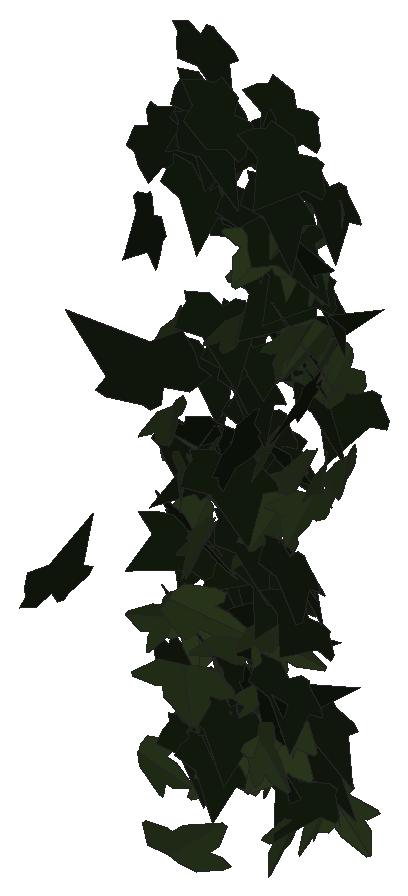
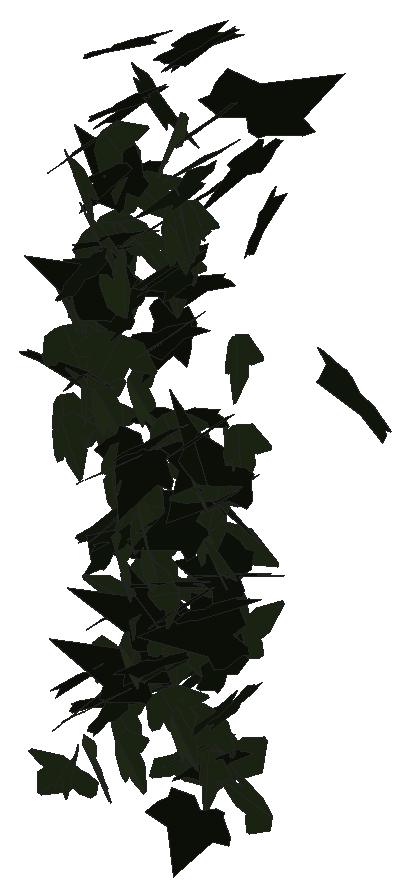
# SketchUp Ruby script. Lengths in inches.
U = 1.inch
M = Sketchup.active_model
def pt(a) = Geom::Point3d.new(a.map { |v| v * U })
def face(e, loops, mat)
  f = e.add_face(loops[0].map { |a| pt(a) })
  loops[1..].each { |l| e.add_face(l.map { |a| pt(a) }).erase! }
  f.material = f.back_material = mat if mat
  f
end
# faces: each face lists its corners as indices into pts; further lists are holes
def faces(e, pts, list, mat = nil) = list.each { |f| face(e, (f[0].is_a?(Array) ? f : [f]).map { |l| l.map { |i| pts[i] } }, mat) }
# xy, xz, yz: faces in a plane at the given z, y or x. An outline is a flat list of corners, or four numbers for a rectangle; further outlines are holes
def ring(l) = l.size == 4 ? [[l[0], l[1]], [l[2], l[1]], [l[2], l[3]], [l[0], l[3]]] : l.each_slice(2).to_a
def flat(e, list, mat, &to3) = list.each { |f| face(e, (f[0].is_a?(Array) ? f : [f]).map { |l| ring(l).map { |u, v| to3.(u, v) } }, mat) }
def xy(e, z, list, mat = nil) = flat(e, list, mat) { |x, y| [x, y, z] }
def xz(e, y, list, mat = nil) = flat(e, list, mat) { |x, z| [x, y, z] }
def yz(e, x, list, mat = nil) = flat(e, list, mat) { |y, z| [x, y, z] }
def lines(e, pts, list) = list.each { |a, b| e.add_line(pt(pts[a]), pt(pts[b])) }
# prism: a flat outline (further loops are holes) pulled along v
def prism(e, loops, v, mat = nil)
  f = face(e, loops, mat); d = Geom::Vector3d.new(v.map { |x| x * U })
  f.pushpull(f.normal.samedirection?(d) ? d.length : -d.length)
end
def box(e, o, s, mat = nil) = prism(e, [[o, [o[0] + s[0], o[1], o[2]], [o[0] + s[0], o[1] + s[1], o[2]], [o[0], o[1] + s[1], o[2]]]], [0, 0, s[2]], mat)
def at(x, y, z, deg = 0) = Geom::Transformation.translation(pt([x, y, z])) * Geom::Transformation.rotation(ORIGIN, Z_AXIS, deg.degrees)
def axes(o, x, y, z) = Geom::Transformation.new([*x, 0, *y, 0, *z, 0, *pt(o).to_a, 1])
def part(name) = M.definitions.add(name)
# library, detail: a bought-in or finely detailed component or shape, given as its bounding box
def library(name, o, s) = part(name).tap { |d| box(d.entities, o, s) }
def detail(e, o, s) = box(e.add_group.entities, o, s)
def put(e, d, t, mat = nil) = e.add_instance(d, t).tap { |i| i.material = mat if mat }
def group(e, t, mat = nil) = e.add_group.tap { |g| g.transformation = t; g.material = mat if mat }.entities
root = M.entities
M.materials.add("1026 AP 7946 SUNNY SIDE UP").color = [254, 231, 186]
M.materials.add("efeu1").color = [18, 25, 13]
M.materials.add("efeu2").color = [43, 57, 29]
c1 = part("ivyleaf_9")
p = [[1.54,2.16,1.25],[1.36,2.04,1.19],[-0.21,0.99,0.68],[-0.71,1.11,0.82],[-0.85,0.86,0.67],[-0.8,0.17,0.21],
  [-0.9,-0.01,0.1],[-0.67,-0.16,-0.02],[-0.08,-0.08,-0.05],[-0.03,-0.6,-0.4],[0.65,-0.88,-0.66],[0.83,-0.6,-0.49],
  [1.29,-0.42,-0.43],[1.8125,-0.07,-0.26],[1.21,0.44,0.15]]
faces(c1.entities,p,[[0,1,2,3,4,5,6,7,8,9,10,11,12,13,14]],"efeu1")
c2 = part("ivyleaf_10")
p = [[0,0.5,-0.03],[-0.0625,2.02,-0.43],[-0.19,2.01,-0.46],[-0.54,1.05,-0.29],[-0.52,0.625,-0.18],[-0.83,0.76,-0.28],
  [-1.16,0.64,-0.33],[-1.15,0.33,-0.24],[-0.77,-0.39,0.02],[-0.3,-0.51,0.16],[0.04,-0.48,0.23],[-0.02,2.01,-0.4375],
  [-0.06,2.01,-0.43],[0.04,-0.49,0.23],[0.67,-0.49,0.14],[1.38,0.36,-0.2],[1.375,0.51,-0.24],[0.81,0.65,-0.19],
  [0.62,0.59,-0.15],[0.6,1.09,-0.28],[0.5,1.23,-0.31]]
faces(c2.entities,p,[[0,1,2,3,4,5,6,7,8,9,10],[11,12,0,13,14,15,16,17,18,19,20]],"efeu2")
put(root,c1,axes([114.58,212.84,282.9],[-0.22038,-0.28928,0.05312],[-0.01341,-0.05491,-0.33106],[0.4623,-0.13949,0.01572]),"1026 AP 7946 SUNNY SIDE UP")
put(root,c1,axes([114.5,211.84,289.67],[0.21549,-0.17371,-0.32569],[-0.19839,0.29264,-0.22098],[0.52993,0.18019,0.04971]),"1026 AP 7946 SUNNY SIDE UP")
put(root,c2,axes([114.73,211.9375,282.02],[-0.07728,-0.11998,-0.35255],[-0.21039,-0.31424,0.13172],[-0.52889,0.14253,-0.00089]),"1026 AP 7946 SUNNY SIDE UP")
put(root,c2,axes([114.29,212.12,279.56],[-0.01905,-0.02116,-0.34342],[0.39995,-0.21662,0.00338],[-0.34016,-0.25351,0.02321]),"1026 AP 7946 SUNNY SIDE UP")
put(root,c2,axes([114.67,212.03,285.18],[-0.06831,-0.33084,-0.06862],[0.03714,0.06211,-0.34304],[0.52878,-0.0471,0.01523]),"1026 AP 7946 SUNNY SIDE UP")
put(root,c1,axes([114.65,212.98,279.74],[0.41387,0.11395,-0.11655],[-0.18573,-0.01156,-0.29349],[-0.1721,0.28651,0.03646]),"1026 AP 7946 SUNNY SIDE UP")
put(root,c1,axes([114.45,212.35,281.24],[0.21928,-0.28954,-0.04148],[-0.01302,0.03886,-0.33071],[0.45912,0.13939,0.01043]),"1026 AP 7946 SUNNY SIDE UP")
put(root,c2,axes([114.71,212.03,286.5625],[0.00107,-0.3309,-0.09887],[0.05564,0.09366,-0.33851],[0.53807,-0.00903,0.0352]),"1026 AP 7946 SUNNY SIDE UP")
put(root,c1,axes([114.49,212.98,290.6],[0.12598,-0.34085,-0.01581],[0.00994,0.01526,-0.36049],[0.53628,0.07979,0.0104]),"1026 AP 7946 SUNNY SIDE UP")
put(root,c1,axes([114.88,212.31,283.09],[-0.42051,-0.13326,0.14679],[-0.08895,-0.17958,-0.28195],[0.29449,-0.24452,0.12444]),"1026 AP 7946 SUNNY SIDE UP")
put(root,c1,axes([114.49,212.39,284.58],[0.27882,-0.24816,-0.14559],[-0.02167,0.15714,-0.3042],[0.44743,0.16225,0.076]),"1026 AP 7946 SUNNY SIDE UP")
put(root,c1,axes([114.36,212.67,282.51],[0.43636,-0.0205,0.1783],[0.2721,-0.00808,-0.28669],[0.03408,0.32702,0.00602]),"1026 AP 7946 SUNNY SIDE UP")
put(root,c1,axes([114.63,211.6875,288.39],[0.09069,-0.16293,-0.33434],[0.35294,-0.24117,0.16489],[-0.44723,-0.22337,0.06233]),"1026 AP 7946 SUNNY SIDE UP")
put(root,c2,axes([114.68,212.53,284.54],[0.33463,0.26404,0.01542],[0.03471,-0.00052,-0.3489],[-0.41426,0.21324,-0.01678]),"1026 AP 7946 SUNNY SIDE UP")
put(root,c1,axes([114.43,212.43,283.3],[0.3313,-0.1951,0.18166],[0.17265,-0.1416,-0.29553],[0.37703,0.23628,-0.02429]),"1026 AP 7946 SUNNY SIDE UP")
put(root,c1,axes([114.66,212.91,285.63],[0.02258,-0.32972,0.04131],[0.0011,-0.04198,-0.34025],[0.52264,0.01434,-0.00107]),"1026 AP 7946 SUNNY SIDE UP")
put(root,c2,axes([114.85,212.47,280.21],[0.01746,-0.29293,-0.13535],[0.04285,0.13019,-0.29971],[0.50192,-0.00093,0.03029]),"1026 AP 7946 SUNNY SIDE UP")
put(root,c1,axes([114.5625,212.5,281.77],[0.10135,-0.21569,0.23287],[0.15687,-0.20583,-0.23159],[0.46704,0.11594,0.02725]),"1026 AP 7946 SUNNY SIDE UP")
put(root,c2,axes([114.88,212.43,283.57],[0.40016,-0.21378,0.02821],[0.0047,-0.04072,-0.34132],[0.33911,0.25283,-0.02855]),"1026 AP 7946 SUNNY SIDE UP")
put(root,c1,axes([114.75,212.33,284.85],[0.47498,0.1731,0.01553],[0.04236,-0.01876,-0.35747],[-0.26977,0.30182,-0.02878]),"1026 AP 7946 SUNNY SIDE UP")
put(root,c2,axes([114.91,212.95,289.11],[0.37554,-0.2474,-0.04236],[0.01544,0.06407,-0.34993],[0.39369,0.23348,0.05413]),"1026 AP 7946 SUNNY SIDE UP")
put(root,c2,axes([115.02,212.94,288.66],[-0.02352,-0.34098,0.04456],[0.00001,-0.04524,-0.35188],[0.54085,-0.01483,0.00194]),"1026 AP 7946 SUNNY SIDE UP")
put(root,c1,axes([115.21,212.23,284.43],[-0.44513,0.16165,-0.08893],[0.09109,-0.07354,-0.33444],[-0.2741,-0.28696,0.03328]),"1026 AP 7946 SUNNY SIDE UP")
put(root,c2,axes([115.09,212.76,288.86],[-0.13165,-0.32957,-0.06683],[0.02391,0.06114,-0.34995],[0.52706,-0.08509,-0.00082]),"1026 AP 7946 SUNNY SIDE UP")
put(root,c1,axes([114.78,212.85,289.51],[0.35689,-0.23602,-0.12388],[-0.0478,0.13238,-0.32971],[0.41279,0.21938,0.06892]),"1026 AP 7946 SUNNY SIDE UP")
put(root,c2,axes([114.97,212.28,281.93],[0.39915,0.2432,-0.00787],[0.0169,-0.02423,-0.36139],[-0.38229,0.25285,-0.0242]),"1026 AP 7946 SUNNY SIDE UP")
put(root,c2,axes([115.1,212.44,284.63],[0.19923,-0.28799,0.12221],[0.03803,-0.12035,-0.32384],[0.48926,0.12662,-0.02459]),"1026 AP 7946 SUNNY SIDE UP")
put(root,c1,axes([115,212.29,280.1],[-0.09276,-0.32021,-0.00661],[0.01114,0.00337,-0.33534],[0.50342,-0.05907,0.0062]),"1026 AP 7946 SUNNY SIDE UP")
put(root,c1,axes([114.83,212.96,288.18],[0.333,-0.269,0.00824],[0.02476,0.00028,-0.35246],[0.42251,0.21199,0.01416]),"1026 AP 7946 SUNNY SIDE UP")
put(root,c1,axes([115,212.92,282.82],[0.0096,-0.3209,0.03841],[0.00361,-0.03906,-0.33088],[0.50831,0.00634,0.00162]),"1026 AP 7946 SUNNY SIDE UP")
put(root,c1,axes([115.04,212.5625,289.57],[-0.1124,-0.31457,0.15233],[0.01649,-0.15464,-0.33063],[0.54751,-0.05992,0.04123]),"1026 AP 7946 SUNNY SIDE UP")
put(root,c1,axes([115.03,212.375,284.77],[0.07041,0.29212,0.19621],[-0.07295,-0.18364,0.30298],[0.54203,-0.06266,0.01529]),"1026 AP 7946 SUNNY SIDE UP")
put(root,c1,axes([115.01,212.29,280.77],[0.04606,-0.29826,0.11801],[0.02103,-0.11549,-0.30941],[0.50291,0.03215,0.00213]),"1026 AP 7946 SUNNY SIDE UP")
put(root,c2,axes([115.23,212.67,280.74],[0.11797,-0.3036,0.07875],[0.01699,-0.07782,-0.32253],[0.49266,0.07538,-0.00773]),"1026 AP 7946 SUNNY SIDE UP")
put(root,c1,axes([115.03,212.96,288.16],[0.13532,-0.31905,-0.09319],[-0.0073,0.09042,-0.33937],[0.52062,0.08419,0.01947]),"1026 AP 7946 SUNNY SIDE UP")
put(root,c2,axes([115.3,212,283.47],[0.0343,-0.3366,0.04549],[-0.00179,-0.04624,-0.34774],[0.5342,0.02146,-0.00409]),"1026 AP 7946 SUNNY SIDE UP")
put(root,c1,axes([114.97,212.69,284.07],[0.4748,-0.1437,0.01439],[0.00109,-0.03282,-0.34337],[0.22715,0.30054,-0.02843]),"1026 AP 7946 SUNNY SIDE UP")
put(root,c2,axes([115.3125,211.49,284.67],[0.23852,-0.25697,-0.16286],[-0.01421,0.17143,-0.29776],[0.47298,0.13474,0.07318]),"1026 AP 7946 SUNNY SIDE UP")
put(root,c1,axes([115.16,212.08,288.93],[-0.04166,-0.3328,0.11502],[-0.01963,-0.1129,-0.34458],[0.55257,-0.0291,-0.00357]),"1026 AP 7946 SUNNY SIDE UP")
put(root,c1,axes([115.375,208.59,284.14],[-0.39717,0.32181,-0.12292],[-0.08975,0.10899,0.42151],[0.53317,0.25807,-0.02061]),"1026 AP 7946 SUNNY SIDE UP")
put(root,c2,axes([115.1875,212.23,284.39],[-0.45676,0.08372,-0.15354],[0.18754,-0.1125,-0.30428],[-0.19346,-0.30672,0.06753]),"1026 AP 7946 SUNNY SIDE UP")
put(root,c2,axes([115.26,212.0625,280.59],[-0.51709,0.07722,-0.08909],[0.12058,-0.05193,-0.34674],[-0.13742,-0.33616,0.03099]),"1026 AP 7946 SUNNY SIDE UP")
put(root,c2,axes([115.44,212.65,281.0625],[-0.1905,-0.27005,0.13265],[-0.0037,-0.13967,-0.30129],[0.47145,-0.11021,0.05123]),"1026 AP 7946 SUNNY SIDE UP")
put(root,c2,axes([115.1875,212.94,283.01],[-0.21967,0.16431,-0.24736],[0.20804,-0.2025,-0.22239],[-0.40881,-0.19135,0.01974]),"1026 AP 7946 SUNNY SIDE UP")
put(root,c1,axes([115.57,212.8125,282.93],[-0.38924,-0.17642,0.11532],[-0.04013,-0.14814,-0.29688],[0.32693,-0.22823,0.10086]),"1026 AP 7946 SUNNY SIDE UP")
put(root,c2,axes([115.41,212.43,289.98],[0.24308,-0.25212,-0.21234],[0.11922,0.24845,-0.25482],[0.49652,0.06378,0.16514]),"1026 AP 7946 SUNNY SIDE UP")
put(root,c2,axes([115.57,212.2,279.92],[0.34474,0.14864,-0.20121],[-0.22389,-0.13766,-0.27222],[-0.31564,0.25999,-0.02666]),"1026 AP 7946 SUNNY SIDE UP")
put(root,c2,axes([115.47,211.82,283.71],[0.12165,-0.28523,0.20019],[0.07665,-0.18979,-0.30557],[0.5387,0.09142,-0.00173]),"1026 AP 7946 SUNNY SIDE UP")
put(root,c1,axes([115.46,212.08,280.02],[-0.09676,-0.30982,0.07186],[0.01044,-0.07408,-0.32516],[0.49986,-0.05842,0.0207]),"1026 AP 7946 SUNNY SIDE UP")
put(root,c2,axes([115.625,212.2,281.82],[-0.28215,-0.26977,-0.02776],[0.04586,0.01108,-0.3332],[0.42359,-0.18089,0.01758]),"1026 AP 7946 SUNNY SIDE UP")
put(root,c2,axes([115.24,211.7,282.48],[-0.1766,-0.07564,-0.33362],[0.51651,0.02522,-0.12345],[0.07728,-0.34143,0.06269]),"1026 AP 7946 SUNNY SIDE UP")
put(root,c2,axes([115.67,212.68,283.27],[0.01768,-0.30032,0.14059],[-0.00036,-0.13826,-0.31038],[0.51981,0.01012,-0.005]),"1026 AP 7946 SUNNY SIDE UP")
put(root,c1,axes([115.42,212.29,281.08],[0.1957,-0.29002,-0.01198],[0.00225,0.01147,-0.325],[0.45629,0.12433,0.00674]),"1026 AP 7946 SUNNY SIDE UP")
put(root,c1,axes([115.64,212.49,286.6],[-0.10076,-0.29176,0.17125],[-0.03286,-0.16712,-0.3084],[0.52827,-0.06605,0.01348]),"1026 AP 7946 SUNNY SIDE UP")
put(root,c1,axes([115.55,212.79,281.72],[0.00188,-0.30727,-0.09968],[0.06674,0.09433,-0.31318],[0.5013,-0.0114,0.04207]),"1026 AP 7946 SUNNY SIDE UP")
put(root,c1,axes([115.67,212.88,285.13],[-0.10425,-0.31558,0.08094],[-0.00105,-0.08187,-0.33229],[0.51205,-0.06442,0.0158]),"1026 AP 7946 SUNNY SIDE UP")
put(root,c1,axes([115.64,212.66,288.46],[-0.01061,-0.33982,0.07516],[0.00772,-0.07498,-0.35053],[0.5471,-0.00553,0.00641]),"1026 AP 7946 SUNNY SIDE UP")
put(root,c1,axes([115.72,212.4,281.36],[-0.14728,-0.24713,0.19154],[0.03181,-0.20014,-0.26275],[0.48657,-0.06172,0.07515]),"1026 AP 7946 SUNNY SIDE UP")
put(root,c1,axes([115.7,211.91,287.2],[-0.13045,-0.32526,-0.09243],[0.0624,0.08044,-0.34484],[0.52608,-0.09019,0.01798]),"1026 AP 7946 SUNNY SIDE UP")
put(root,c2,axes([115.89,212.6,283.73],[0.14154,-0.31567,-0.05351],[-0.00775,0.05072,-0.33774],[0.50252,0.08969,0.00986]),"1026 AP 7946 SUNNY SIDE UP")
put(root,c1,axes([115.67,212.43,282.125],[-0.22308,0.19174,0.24342],[0.23533,-0.18165,0.24449],[0.41507,0.20603,-0.00779]),"1026 AP 7946 SUNNY SIDE UP")
put(root,c1,axes([115.7,211.63,290.77],[0.00157,-0.3656,0.01363],[-0.00124,-0.01531,-0.37673],[0.57538,0.00097,-0.00085]),"1026 AP 7946 SUNNY SIDE UP")
put(root,c1,axes([115.93,212.18,280.9],[-0.27549,-0.17461,0.25612],[-0.09371,-0.26273,-0.23398],[0.46972,-0.15482,0.10353]),"1026 AP 7946 SUNNY SIDE UP")
put(root,c1,axes([115.85,212.27,280.63],[-0.09645,0.01977,0.33532],[-0.04787,-0.32999,0.01281],[0.51033,-0.02722,0.06458]),"1026 AP 7946 SUNNY SIDE UP")
put(root,c2,axes([116,211.91,284.83],[-0.12862,-0.32027,0.07906],[0.00526,-0.08175,-0.34019],[0.51849,-0.07862,0.02307]),"1026 AP 7946 SUNNY SIDE UP")
put(root,c1,axes([115.9,212.61,284.78],[0.46673,0.02472,-0.16165],[-0.24289,-0.03385,-0.30645],[-0.05915,0.3341,-0.0171]),"1026 AP 7946 SUNNY SIDE UP")
put(root,c1,axes([115.8,212.28,283.68],[0.05575,-0.33782,-0.03487],[-0.00761,0.0316,-0.34974],[0.5335,0.03575,-0.00134]),"1026 AP 7946 SUNNY SIDE UP")
put(root,c2,axes([115.8,210.85,279.1875],[-0.43923,-0.15837,0.20532],[0.27643,0.09583,0.33135],[-0.29103,0.33004,0.00486]),"1026 AP 7946 SUNNY SIDE UP")
put(root,c1,axes([115.93,212.27,286.49],[-0.18511,-0.31883,-0.03189],[0.02306,0.02565,-0.34994],[0.50289,-0.11854,0.00431]),"1026 AP 7946 SUNNY SIDE UP")
put(root,c2,axes([116.01,212.48,283.59],[-0.03589,-0.30003,0.12337],[0.08891,-0.12358,-0.30427],[0.50112,0.00044,0.06282]),"1026 AP 7946 SUNNY SIDE UP")
put(root,c1,axes([116.14,211.54,290.59],[-0.27042,-0.2164,0.26198],[-0.2138,-0.21738,-0.2852],[0.48116,-0.21821,0.02051]),"1026 AP 7946 SUNNY SIDE UP")
put(root,c2,axes([116.32,212.29,287.91],[0.34714,-0.1433,-0.25196],[-0.36297,0.08728,-0.26772],[0.25679,0.31708,-0.0378]),"1026 AP 7946 SUNNY SIDE UP")
put(root,c2,axes([116.14,211.67,287.28],[-0.07439,-0.34948,-0.04904],[0.01822,0.04446,-0.36301],[0.55388,-0.0484,0.00536]),"1026 AP 7946 SUNNY SIDE UP")
put(root,c1,axes([115.84,212.79,284.84],[0.2303,-0.26888,-0.13905],[0.03417,0.1576,-0.30162],[0.47076,0.1201,0.08992]),"1026 AP 7946 SUNNY SIDE UP")
put(root,c2,axes([116.13,212.49,283.47],[0.26643,-0.28288,0.04833],[0.00795,-0.0534,-0.33919],[0.45123,0.16797,-0.02256]),"1026 AP 7946 SUNNY SIDE UP")
put(root,c2,axes([116.12,212.43,284.16],[-0.12245,-0.26821,-0.19946],[0.12294,0.17675,-0.28585],[0.50396,-0.10828,0.02127]),"1026 AP 7946 SUNNY SIDE UP")
put(root,c1,axes([116.02,211.69,284.94],[-0.18233,-0.29627,-0.14831],[0.10751,0.12583,-0.32659],[0.50548,-0.13363,0.01597]),"1026 AP 7946 SUNNY SIDE UP")
put(root,c2,axes([116.21,212.62,280.03],[0.06433,-0.3097,0.07393],[-0.00042,-0.07416,-0.3221],[0.5005,0.03974,-0.00978]),"1026 AP 7946 SUNNY SIDE UP")
put(root,c2,axes([116.22,212.76,283.22],[0.17121,-0.30566,-0.05483],[-0.02033,0.05004,-0.33395],[0.48697,0.10956,0.00533]),"1026 AP 7946 SUNNY SIDE UP")
put(root,c1,axes([115.76,212.25,281.9],[0.14453,0.02541,0.35255],[0.53309,-0.06053,-0.08958],[0.08194,0.34899,-0.03909]),"1026 AP 7946 SUNNY SIDE UP")
put(root,c1,axes([116.36,212.03,290.13],[-0.42947,0.16175,-0.16575],[0.183,-0.11873,-0.32533],[-0.30973,-0.29442,0.03761]),"1026 AP 7946 SUNNY SIDE UP")
put(root,c1,axes([115.98,211.19,290.5],[0.10536,-0.34869,-0.04692],[0.00165,0.04455,-0.3654],[0.55253,0.06635,0.01004]),"1026 AP 7946 SUNNY SIDE UP")
put(root,c1,axes([116.02,212.15,286.23],[0.02462,-0.34362,0.06673],[0.01343,-0.0664,-0.35471],[0.55024,0.017,0.00567]),"1026 AP 7946 SUNNY SIDE UP")
put(root,c1,axes([116.12,211.54,281.22],[-0.16106,-0.33639,0.00899],[0.00916,-0.01289,-0.36221],[0.52913,-0.10217,0.00901]),"1026 AP 7946 SUNNY SIDE UP")
put(root,c2,axes([116.18,212.59,281.53],[0.16795,-0.25146,0.17375],[0.09534,-0.159,-0.28233],[0.46774,0.1227,-0.00484]),"1026 AP 7946 SUNNY SIDE UP")
put(root,c2,axes([116.35,212.35,284.15],[-0.25227,-0.2762,0.17514],[-0.05062,-0.17689,-0.3254],[0.50875,-0.15455,0.05447]),"1026 AP 7946 SUNNY SIDE UP")
put(root,c2,axes([116.3,210.37,282.34],[-0.58209,-0.15484,-0.01178],[0.03674,-0.0286,-0.41194],[0.24125,-0.36923,0.0343]),"1026 AP 7946 SUNNY SIDE UP")
put(root,c1,axes([116.25,212.79,290.17],[-0.22223,-0.27482,0.17472],[-0.06742,-0.16923,-0.31738],[0.5046,-0.14364,0.03454]),"1026 AP 7946 SUNNY SIDE UP")
put(root,c2,axes([116.3,212.48,284.54],[-0.18727,-0.2919,-0.09384],[0.05974,0.08107,-0.32428],[0.47631,-0.12493,0.00378]),"1026 AP 7946 SUNNY SIDE UP")
put(root,c2,axes([116.33,212.04,281.65],[0.00404,0.18807,-0.28793],[0.02051,0.28031,0.19533],[0.5307,-0.01227,-0.00536]),"1026 AP 7946 SUNNY SIDE UP")
put(root,c2,axes([116.36,211.95,281.37],[-0.01427,-0.274,0.18412],[0.04764,-0.18028,-0.28176],[0.51353,0.00911,0.03126]),"1026 AP 7946 SUNNY SIDE UP")
put(root,c2,axes([116.49,211.98,288.46],[-0.32963,-0.17098,0.23159],[-0.07498,-0.25558,-0.2465],[0.43897,-0.17205,0.1318]),"1026 AP 7946 SUNNY SIDE UP")
put(root,c2,axes([116.32,212.71,286.34],[-0.40872,-0.19956,-0.10814],[0.18936,0.01059,-0.33146],[0.29877,-0.27971,0.06213]),"1026 AP 7946 SUNNY SIDE UP")
put(root,c2,axes([116.375,211.96,282.45],[-0.13446,-0.2698,-0.17854],[0.11763,0.156,-0.28988],[0.48896,-0.11172,0.02064]),"1026 AP 7946 SUNNY SIDE UP")
put(root,c2,axes([116.44,212.08,285.35],[0.14124,-0.30955,0.12017],[0.03757,-0.11631,-0.3326],[0.51977,0.09252,-0.00861]),"1026 AP 7946 SUNNY SIDE UP")
put(root,c2,axes([116.37,212.5,286.92],[-0.039,-0.27475,-0.22374],[0.03567,-0.21698,0.28087],[-0.54801,0.00543,0.0342]),"1026 AP 7946 SUNNY SIDE UP")
put(root,c1,axes([116.5,212.35,283.05],[-0.2915,-0.25978,0.05256],[-0.03074,-0.05049,-0.32879],[0.4156,-0.18594,0.01255]),"1026 AP 7946 SUNNY SIDE UP")
put(root,c1,axes([116.14,212.3,280.99],[0.08505,-0.00661,0.36191],[0.54936,0.03907,-0.05442],[-0.05915,0.35332,0.01488]),"1026 AP 7946 SUNNY SIDE UP")
put(root,c1,axes([116.59,212.27,287.6],[-0.36354,-0.22439,0.14805],[-0.03558,-0.1746,-0.31658],[0.41857,-0.20973,0.10167]),"1026 AP 7946 SUNNY SIDE UP")
put(root,c1,axes([116.24,212.49,286.85],[0.3027,-0.26109,0.10857],[0.07245,-0.09854,-0.3341],[0.43764,0.1969,-0.01978]),"1026 AP 7946 SUNNY SIDE UP")
put(root,c1,axes([116.36,212.72,283.13],[0.11816,-0.27756,0.16679],[0.07314,-0.15675,-0.29713],[0.50119,0.08831,0.00404]),"1026 AP 7946 SUNNY SIDE UP")
put(root,c1,axes([116.67,212.57,287.83],[-0.32635,-0.24641,0.12373],[-0.04549,-0.13182,-0.32711],[0.4296,-0.20115,0.05935]),"1026 AP 7946 SUNNY SIDE UP")
put(root,c1,axes([116.73,210.87,285.89],[-0.03286,0.0321,-0.41799],[-0.38491,0.32382,0.04126],[0.51166,0.24566,0.00419]),"1026 AP 7946 SUNNY SIDE UP")
put(root,c1,axes([116.43,211.84,281.18],[-0.07393,0.01427,0.34833],[0.17853,-0.32084,0.02834],[0.50116,0.11639,0.04129]),"1026 AP 7946 SUNNY SIDE UP")
put(root,c2,axes([116.26,212.23,282.08],[-0.01998,0.03127,0.36672],[0.56156,-0.0034,0.01343],[0.00712,0.356,-0.02999]),"1026 AP 7946 SUNNY SIDE UP")
put(root,c1,axes([116.56,212.31,283.41],[0.03901,-0.32786,0.08158],[-0.00972,-0.08169,-0.33898],[0.53096,0.02259,-0.0122]),"1026 AP 7946 SUNNY SIDE UP")
put(root,c1,axes([117.13,208.74,287.95],[0.08011,0.08408,0.43915],[-0.6809,-0.01915,0.05716],[0.04615,-0.42841,0.08102]),"1026 AP 7946 SUNNY SIDE UP")
put(root,c1,axes([116.59,212.05,288.73],[0.04839,-0.2835,-0.22652],[0.02183,0.21986,-0.29088],[0.56217,0.01587,0.0308]),"1026 AP 7946 SUNNY SIDE UP")
put(root,c2,axes([116.77,211.97,281.04],[0.5185,-0.08056,-0.00787],[-0.02248,-0.0284,-0.3484],[0.12518,0.3286,-0.02999]),"1026 AP 7946 SUNNY SIDE UP")
put(root,c2,axes([116.86,211.71,280.77],[0.31992,0.20166,-0.19645],[-0.18059,-0.15563,-0.29493],[-0.39865,0.23233,-0.02405]),"1026 AP 7946 SUNNY SIDE UP")
put(root,c2,axes([116.88,212.07,289.08],[-0.09087,-0.29389,0.18029],[0.01049,-0.18009,-0.30743],[0.53908,-0.04603,0.03637]),"1026 AP 7946 SUNNY SIDE UP")
put(root,c1,axes([116.73,212.32,280.21],[-0.08043,-0.20406,0.2667],[0.01585,-0.26398,-0.21291],[0.51952,-0.02354,0.04779]),"1026 AP 7946 SUNNY SIDE UP")
put(root,c1,axes([116.83,212.71,280.47],[-0.18895,-0.24172,0.17538],[-0.03646,-0.17695,-0.27451],[0.4647,-0.11217,0.04977]),"1026 AP 7946 SUNNY SIDE UP")
put(root,c2,axes([116.87,212.48,287.97],[0.40478,-0.23718,-0.0007],[-0.02603,-0.01895,-0.35978],[0.37203,0.25673,-0.02441]),"1026 AP 7946 SUNNY SIDE UP")
put(root,c1,axes([116.68,212.73,285.96],[0.14581,-0.31725,0.03971],[0.00433,-0.04121,-0.34062],[0.50284,0.09235,-0.00858]),"1026 AP 7946 SUNNY SIDE UP")
put(root,c2,axes([116.91,212.25,285.11],[0.07058,-0.30802,0.15098],[0.05187,-0.14498,-0.32133],[0.53504,0.05468,0.01123]),"1026 AP 7946 SUNNY SIDE UP")
put(root,c1,axes([116.69,212.93,287.38],[0.08394,-0.2851,0.1834],[0.06751,-0.17465,-0.2997],[0.52554,0.06797,0.00921]),"1026 AP 7946 SUNNY SIDE UP")
put(root,c1,axes([116.62,212.41,286.86],[0.06679,-0.04284,0.36121],[0.53214,0.10695,-0.02813],[-0.16045,0.33686,0.05707]),"1026 AP 7946 SUNNY SIDE UP")
put(root,c2,axes([116.93,212.89,279.7],[-0.09585,0.30429,-0.03479],[-0.03146,-0.04007,-0.3187],[-0.48068,-0.05805,0.0278]),"1026 AP 7946 SUNNY SIDE UP")
put(root,c2,axes([117.06,212.79,286.24],[-0.27035,-0.277,0.09396],[-0.03205,-0.09602,-0.3348],[0.45822,-0.17015,0.03202]),"1026 AP 7946 SUNNY SIDE UP")
put(root,c2,axes([117,212.71,288.88],[0.36084,-0.25076,-0.06437],[-0.04825,0.05461,-0.34956],[0.40294,0.2311,0.01579]),"1026 AP 7946 SUNNY SIDE UP")
put(root,c2,axes([117,212.5625,286.79],[-0.01178,-0.30962,0.1459],[0.04016,-0.14352,-0.31875],[0.53502,0.00396,0.02714]),"1026 AP 7946 SUNNY SIDE UP")
put(root,c1,axes([116.83,211.96,281.73],[-0.05061,-0.33824,0.09066],[0.00128,-0.09038,-0.35043],[0.55032,-0.03089,0.00915]),"1026 AP 7946 SUNNY SIDE UP")
put(root,c1,axes([116.64,212.125,288.43],[0.06356,-0.09599,0.35124],[0.27375,-0.29409,-0.10811],[0.48597,0.17822,0.01496]),"1026 AP 7946 SUNNY SIDE UP")
put(root,c2,axes([117.01,212.36,279.54],[0.28582,-0.27742,0.02795],[-0.00001,-0.03427,-0.34134],[0.43855,0.18081,-0.01823]),"1026 AP 7946 SUNNY SIDE UP")
put(root,c1,axes([116.83,211.73,289.51],[0.00063,-0.35463,0.02047],[0.00361,-0.02189,-0.36545],[0.55867,0.00054,0.00234]),"1026 AP 7946 SUNNY SIDE UP")
put(root,c2,axes([117.09,212.8,284.79],[-0.02438,-0.33108,0.03681],[0.00745,-0.03787,-0.3416],[0.52388,-0.01487,0.00657]),"1026 AP 7946 SUNNY SIDE UP")
put(root,c2,axes([117.13,212,284.625],[-0.19897,-0.29288,0.11724],[-0.01812,-0.12005,-0.32742],[0.49469,-0.1222,0.03516]),"1026 AP 7946 SUNNY SIDE UP")
put(root,c1,axes([116.74,212.15,287.17],[0.22358,-0.24814,0.19229],[0.12674,-0.17037,-0.29535],[0.47289,0.16298,-0.01176]),"1026 AP 7946 SUNNY SIDE UP")
put(root,c1,axes([116.91,212.56,280.97],[0.06678,-0.30995,-0.07842],[0.02017,0.07662,-0.32101],[0.50079,0.03824,0.02339]),"1026 AP 7946 SUNNY SIDE UP")
put(root,c1,axes([116.9,212.37,280.51],[0.19874,-0.28337,-0.11499],[-0.04119,0.10854,-0.3184],[0.47619,0.12765,0.02045]),"1026 AP 7946 SUNNY SIDE UP")
put(root,c2,axes([117.18,211.74,287.41],[-0.04659,-0.38232,0.07878],[-0.00976,-0.0784,-0.3955],[0.61367,-0.03027,-0.00031]),"1026 AP 7946 SUNNY SIDE UP")
put(root,c1,axes([116.94,212.69,289.2],[0.00488,-0.34289,0.0951],[0.00219,-0.09425,-0.3538],[0.55915,0.00336,0.00056]),"1026 AP 7946 SUNNY SIDE UP")
put(root,c1,axes([117.18,211.99,280.23],[-0.2623,-0.2757,0.11122],[-0.06057,-0.10446,-0.33194],[0.46251,-0.17003,0.0196]),"1026 AP 7946 SUNNY SIDE UP")
put(root,c2,axes([117.17,211.49,279.71],[0.02251,-0.28875,0.14927],[0.06793,-0.14366,-0.29683],[0.5046,0.03222,0.0333]),"1026 AP 7946 SUNNY SIDE UP")
put(root,c1,axes([117.1875,211.65,290.27],[-0.29866,-0.27219,0.15723],[-0.03979,-0.1664,-0.33575],[0.49027,-0.17932,0.06853]),"1026 AP 7946 SUNNY SIDE UP")
put(root,c1,axes([117.16,212.9375,285.9],[-0.42484,-0.16853,-0.11135],[0.22094,-0.03238,-0.31281],[0.22312,-0.28884,0.09774]),"1026 AP 7946 SUNNY SIDE UP")
put(root,c2,axes([116.79,211.39,280.93],[0.11245,0.01082,0.39909],[0.53178,-0.19399,-0.05988],[0.29739,0.3428,-0.04383]),"1026 AP 7946 SUNNY SIDE UP")
put(root,c2,axes([117.26,212.01,287.3125],[-0.07847,-0.2648,0.23598],[-0.00642,-0.23243,-0.27727],[0.55205,-0.04034,0.03032]),"1026 AP 7946 SUNNY SIDE UP")
put(root,c2,axes([117.24,212.65,285.02],[-0.00613,-0.33448,-0.05786],[0.02312,0.05405,-0.34399],[0.53232,-0.0062,0.01427]),"1026 AP 7946 SUNNY SIDE UP")
put(root,c2,axes([117.22,212.17,285.08],[0.07435,-0.31832,-0.1082],[0.0324,0.10682,-0.32901],[0.52519,0.03848,0.03562]),"1026 AP 7946 SUNNY SIDE UP")
put(root,c1,axes([117.16,211.94,282.84],[-0.21589,-0.22839,0.24119],[0.0102,-0.25705,-0.25452],[0.51564,-0.09054,0.10602]),"1026 AP 7946 SUNNY SIDE UP")
put(root,c2,axes([117.27,212.59,286.7],[0.33731,-0.26964,0.00761],[-0.01346,-0.0182,-0.35458],[0.424,0.21393,-0.01732]),"1026 AP 7946 SUNNY SIDE UP")
put(root,c1,axes([117.24,211.97,286.49],[-0.19897,-0.02582,-0.33984],[0.34368,-0.27149,-0.0661],[-0.39032,-0.2259,0.11504]),"1026 AP 7946 SUNNY SIDE UP")
put(root,c2,axes([117.03,212.77,279.45],[0.37698,0.07541,0.19029],[0.27604,0.05607,-0.25859],[-0.14777,0.29715,0.00241]),"1026 AP 7946 SUNNY SIDE UP")
